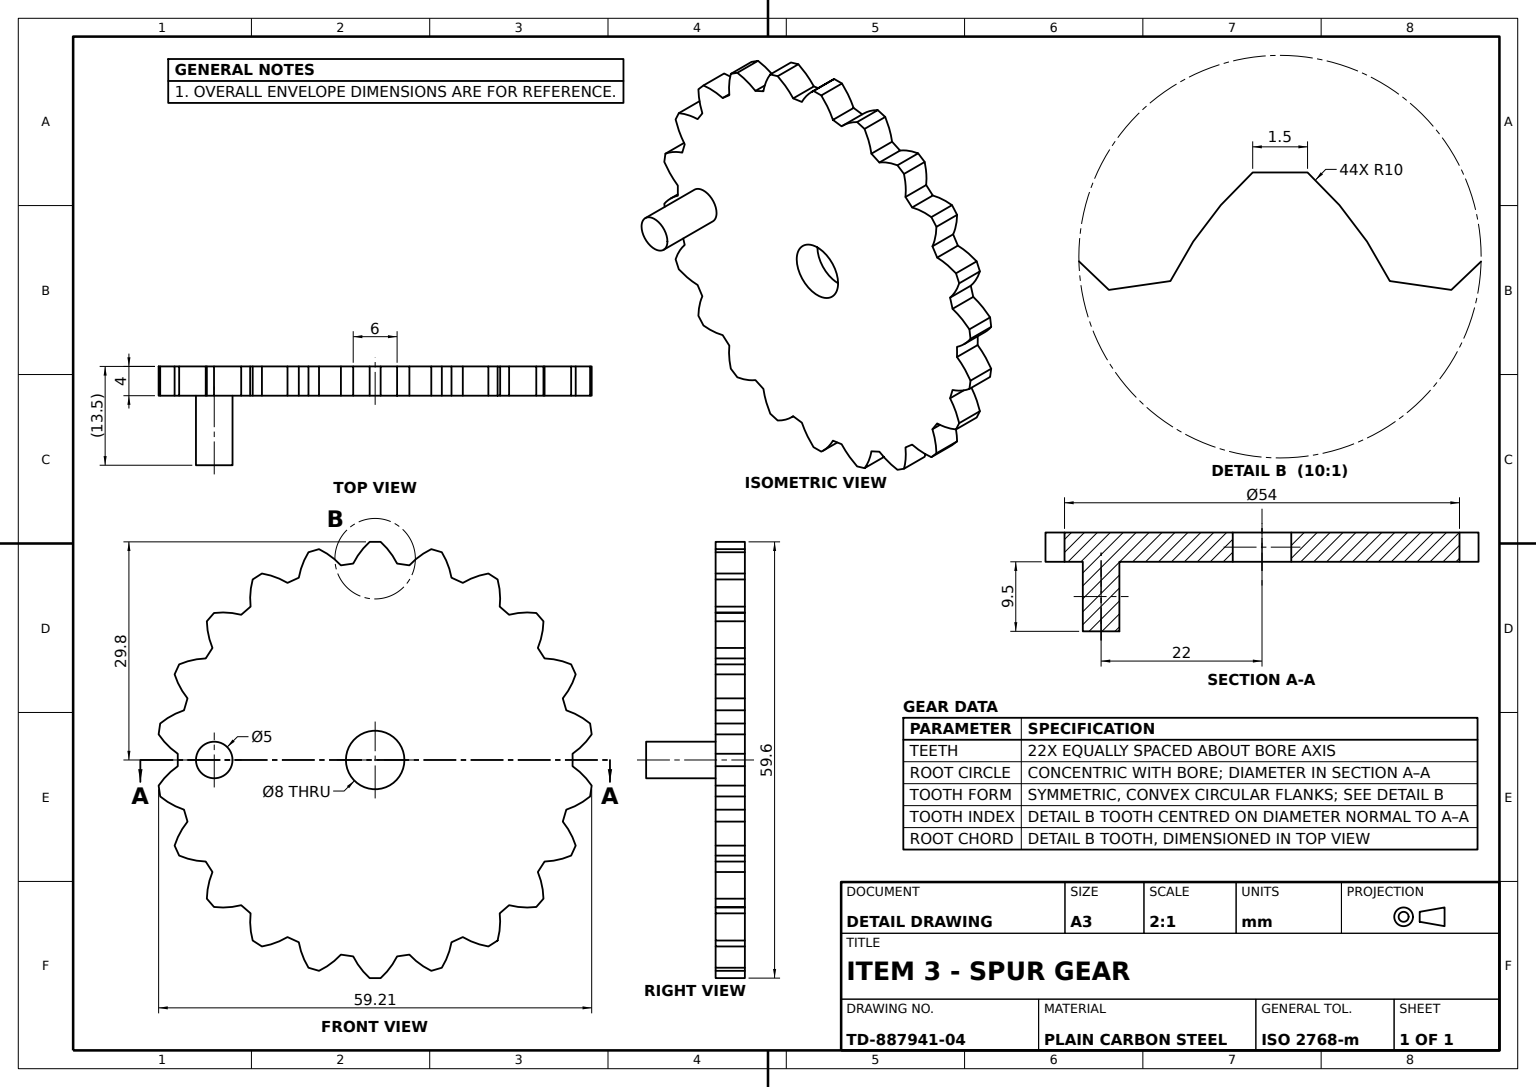
solid
v1 (-3,-26.832816,-4)
v2 (-3,-26.832816,0)
e1 v1 v2 LINE
v3 (-0.75,-29.8,-4)
e2 v3 v1 CIRCLE(AX(P(5.95383,-22.379848,-4),D(0,0,-1),D(1,0,0)),10)
v4 (-0.75,-29.8,0)
e3 v3 v4 LINE
e4 v4 v2 CIRCLE(AX(P(5.95383,-22.379848,0),D(0,0,-1),D(1,0,0)),10)
face CYL(AX(P(5.95383,-22.379848,-4),D(0,0,1),D(1,0,0)),10) [-e1 -e2 e3 e4]
v5 (-15.480156,-25.474836,0)
v6 (-16.742037,-24.663875,0)
e5 v5 v6 LINE
v7 (-16.742037,-24.663875,-4)
e6 v7 v6 LINE
v8 (-15.480156,-25.474836,-4)
e7 v8 v7 LINE
e8 v8 v5 LINE
face PLANE(AX(P(-16.111096,-25.069355,-4),D(0.540640817,0.841253533,0),D(-0.841253533,0.540640817,0))) rev [e5 -e6 -e7 e8]
v9 (-0.75,29.8,0)
v10 (-3,26.832816,0)
e9 v9 v10 CIRCLE(AX(P(5.95383,22.379848,0),D(0,0,1),D(1,0,0)),10)
v11 (-0.75,29.8,-4)
e10 v11 v9 LINE
v12 (-3,26.832816,-4)
e11 v11 v12 CIRCLE(AX(P(5.95383,22.379848,-4),D(0,0,1),D(1,0,0)),10)
e12 v12 v10 LINE
face CYL(AX(P(5.95383,22.379848,-4),D(0,0,1),D(1,0,0)),10) [-e9 -e10 e11 e12]
v13 (22.030192,20.081662,0)
v14 (23.012483,18.948038,0)
e13 v13 v14 LINE
v15 (23.012483,18.948038,-4)
e14 v15 v14 LINE
v16 (22.030192,20.081662,-4)
e15 v16 v15 LINE
e16 v16 v13 LINE
face PLANE(AX(P(22.521337,19.51485,-4),D(-0.755749574,-0.654860734,0),D(0.654860734,-0.755749574,0))) rev [e13 -e14 -e15 e16]
v17 (-23.012483,18.948038,-4)
v18 (-22.243471,15.304509,-4)
e17 v17 v18 CIRCLE(AX(P(-13.014631,19.155288,-4),D(0,0,1),D(1,0,0)),10)
v19 (-22.243471,15.304509,0)
e18 v18 v19 LINE
v20 (-23.012483,18.948038,0)
e19 v20 v19 CIRCLE(AX(P(-13.014631,19.155288,0),D(0,0,1),D(1,0,0)),10)
e20 v17 v20 LINE
face CYL(AX(P(-13.014631,19.155288,-4),D(0,0,1),D(1,0,0)),10) [e17 e18 -e19 -e20]
v21 (-7.67601,28.80419,0)
v22 (-4.681199,26.591096,0)
e21 v21 v22 CIRCLE(AX(P(-12.01779,19.795919,0),D(0,0,-1),D(1,0,0)),10)
v23 (-4.681199,26.591096,-4)
e22 v23 v22 LINE
v24 (-7.67601,28.80419,-4)
e23 v24 v23 CIRCLE(AX(P(-12.01779,19.795919,-4),D(0,0,-1),D(1,0,0)),10)
e24 v24 v21 LINE
face CYL(AX(P(-12.01779,19.795919,-4),D(0,0,1),D(1,0,0)),10) [e21 -e22 -e23 e24]
v25 (-19.5,0,9.5)
v26 (-19.5,0,0)
e25 v25 v26 LINE
v27 (-24.5,0,9.5)
e26 v27 v25 CIRCLE(AX(P(-22,0,9.5),D(0,0,1),D(1,0,0)),2.5)
v28 (-24.5,0,0)
e27 v27 v28 LINE
e28 v28 v26 CIRCLE(AX(P(-22,0,0),D(0,0,1),D(1,0,0)),2.5)
face CYL(AX(P(-22,0,9.5),D(0,0,-1),D(-1,0,0)),2.5) [-e25 -e26 e27 e28]
v29 (-15.480156,25.474836,-4)
v30 (-15.480156,25.474836,0)
e29 v29 v30 LINE
v31 (-11.983155,24.195123,0)
e30 v30 v31 CIRCLE(AX(P(-17.10814,15.608242,0),D(0,0,-1),D(1,0,0)),10)
v32 (-11.983155,24.195123,-4)
e31 v32 v31 LINE
e32 v29 v32 CIRCLE(AX(P(-17.10814,15.608242,-4),D(0,0,-1),D(1,0,0)),10)
face CYL(AX(P(-17.10814,15.608242,-4),D(0,0,1),D(1,0,0)),10) [e29 e30 -e31 -e32]
v33 (10.438157,24.9007,-4)
v34 (10.438157,24.9007,0)
e33 v33 v34 LINE
v35 (11.983155,24.195123,0)
e34 v35 v34 CIRCLE(AX(P(0,0,0),D(0,0,1),D(1,0,0)),27)
v36 (11.983155,24.195123,-4)
e35 v36 v35 LINE
e36 v36 v33 CIRCLE(AX(P(0,0,-4),D(0,0,1),D(1,0,0)),27)
face CYL(AX(P(0,0,-4),D(0,0,1),D(1,0,0)),27) [e33 -e34 -e35 e36]
v37 (23.012483,-18.948038,-4)
v38 (22.243471,-15.304509,-4)
e37 v37 v38 CIRCLE(AX(P(13.014631,-19.155288,-4),D(0,0,1),D(1,0,0)),10)
v39 (22.243471,-15.304509,0)
e38 v38 v39 LINE
v40 (23.012483,-18.948038,0)
e39 v40 v39 CIRCLE(AX(P(13.014631,-19.155288,0),D(0,0,1),D(1,0,0)),10)
e40 v37 v40 LINE
face CYL(AX(P(13.014631,-19.155288,-4),D(0,0,1),D(1,0,0)),10) [e37 e38 -e39 -e40]
v41 (-26.986641,-0.849244,-4)
v42 (-26.986641,-0.849244,0)
e41 v41 v42 LINE
v43 (-29.603415,-3.498616,-4)
e42 v43 v41 CIRCLE(AX(P(-21.304735,-9.078213,-4),D(0,0,-1),D(1,0,0)),10)
v44 (-29.603415,-3.498616,0)
e43 v43 v44 LINE
e44 v44 v42 CIRCLE(AX(P(-21.304735,-9.078213,0),D(0,0,-1),D(1,0,0)),10)
face CYL(AX(P(-21.304735,-9.078213,-4),D(0,0,1),D(1,0,0)),10) [-e41 -e42 e43 e44]
v45 (-26.795472,-13.061591,0)
v46 (-27.418595,-11.697143,0)
e45 v45 v46 LINE
v47 (-27.418595,-11.697143,-4)
e46 v47 v46 LINE
v48 (-26.795472,-13.061591,-4)
e47 v48 v47 LINE
e48 v48 v45 LINE
face PLANE(AX(P(-27.107033,-12.379367,-4),D(0.909631995,0.415415013,0),D(-0.415415013,0.909631995,0))) rev [e45 -e46 -e47 e48]
e49 v26 v28 CIRCLE(AX(P(-22,0,0),D(0,0,1),D(1,0,0)),2.5)
e50 v25 v27 CIRCLE(AX(P(-22,0,9.5),D(0,0,1),D(1,0,0)),2.5)
face CYL(AX(P(-22,0,9.5),D(0,0,-1),D(-1,0,0)),2.5) [e25 e49 -e27 -e50]
v49 (7.67601,-28.80419,-4)
v50 (7.67601,-28.80419,0)
e51 v49 v50 LINE
v51 (4.681199,-26.591096,0)
e52 v50 v51 CIRCLE(AX(P(12.01779,-19.795919,0),D(0,0,-1),D(1,0,0)),10)
v52 (4.681199,-26.591096,-4)
e53 v52 v51 LINE
e54 v49 v52 CIRCLE(AX(P(12.01779,-19.795919,-4),D(0,0,-1),D(1,0,0)),10)
face CYL(AX(P(12.01779,-19.795919,-4),D(0,0,1),D(1,0,0)),10) [e51 e52 -e53 -e54]
v53 (29.603415,-3.498616,0)
v54 (29.389943,-4.983348,0)
e55 v53 v54 LINE
v55 (29.389943,-4.983348,-4)
e56 v55 v54 LINE
v56 (29.603415,-3.498616,-4)
e57 v56 v55 LINE
e58 v56 v53 LINE
face PLANE(AX(P(29.496679,-4.240982,-4),D(-0.989821442,0.142314838,0),D(-0.142314838,-0.989821442,0))) rev [e55 -e56 -e57 e58]
v57 (-22.030192,-20.081662,0)
v58 (-18.314307,-19.839006,0)
e59 v57 v58 CIRCLE(AX(P(-20.81249,-10.156079,0),D(0,0,1),D(1,0,0)),10)
v59 (-22.030192,-20.081662,-4)
e60 v59 v57 LINE
v60 (-18.314307,-19.839006,-4)
e61 v59 v60 CIRCLE(AX(P(-20.81249,-10.156079,-4),D(0,0,1),D(1,0,0)),10)
e62 v60 v58 LINE
face CYL(AX(P(-20.81249,-10.156079,-4),D(0,0,1),D(1,0,0)),10) [-e59 -e60 e61 e62]
v61 (22.030192,-20.081662,-4)
v62 (18.314307,-19.839006,-4)
e63 v61 v62 CIRCLE(AX(P(20.81249,-10.156079,-4),D(0,0,-1),D(1,0,0)),10)
v63 (22.030192,-20.081662,0)
e64 v61 v63 LINE
v64 (18.314307,-19.839006,0)
e65 v63 v64 CIRCLE(AX(P(20.81249,-10.156079,0),D(0,0,-1),D(1,0,0)),10)
e66 v62 v64 LINE
face CYL(AX(P(20.81249,-10.156079,-4),D(0,0,1),D(1,0,0)),10) [-e63 e64 e65 -e66]
v65 (27,0,-4)
v66 (26.986641,0.849244,-4)
e67 v65 v66 CIRCLE(AX(P(0,0,-4),D(0,0,1),D(1,0,0)),27)
v67 (26.986641,0.849244,0)
e68 v66 v67 LINE
v68 (27,0,0)
e69 v68 v67 CIRCLE(AX(P(0,0,0),D(0,0,1),D(1,0,0)),27)
e70 v65 v68 LINE
face CYL(AX(P(0,0,-4),D(0,0,1),D(1,0,0)),27) [e67 e68 -e69 -e70]
v69 (-22.030192,20.081662,-4)
e71 v17 v69 LINE
v70 (-22.030192,20.081662,0)
e72 v20 v70 LINE
e73 v69 v70 LINE
face PLANE(AX(P(-22.521337,19.51485,-4),D(0.755749574,-0.654860734,0),D(0.654860734,0.755749574,0))) rev [-e71 e20 e72 -e73]
v71 (27.418595,11.697143,-4)
v72 (27.418595,11.697143,0)
e74 v71 v72 LINE
v73 (25.654233,8.417859,0)
e75 v72 v73 CIRCLE(AX(P(17.884115,14.712719,0),D(0,0,-1),D(1,0,0)),10)
v74 (25.654233,8.417859,-4)
e76 v74 v73 LINE
e77 v71 v74 CIRCLE(AX(P(17.884115,14.712719,-4),D(0,0,-1),D(1,0,0)),10)
face CYL(AX(P(17.884115,14.712719,-4),D(0,0,1),D(1,0,0)),10) [e74 e75 -e76 -e77]
v75 (-17.030676,-20.951279,-4)
e78 v60 v75 CIRCLE(AX(P(0,0,-4),D(0,0,1),D(1,0,0)),27)
v76 (-17.030676,-20.951279,0)
e79 v75 v76 LINE
e80 v58 v76 CIRCLE(AX(P(0,0,0),D(0,0,1),D(1,0,0)),27)
face CYL(AX(P(0,0,-4),D(0,0,1),D(1,0,0)),27) [-e62 e78 e79 -e80]
v77 (-16.742037,24.663875,-4)
v78 (-16.742037,24.663875,0)
e81 v77 v78 LINE
e82 v78 v30 LINE
e83 v77 v29 LINE
face PLANE(AX(P(-16.111096,25.069355,-4),D(0.540640817,-0.841253533,0),D(0.841253533,0.540640817,0))) rev [e81 e82 -e29 -e83]
v79 (-26.795472,13.061591,-4)
v80 (-23.161743,13.87565,-4)
e84 v79 v80 CIRCLE(AX(P(-22.830736,3.88113,-4),D(0,0,-1),D(1,0,0)),10)
v81 (-26.795472,13.061591,0)
e85 v79 v81 LINE
v82 (-23.161743,13.87565,0)
e86 v81 v82 CIRCLE(AX(P(-22.830736,3.88113,0),D(0,0,-1),D(1,0,0)),10)
e87 v80 v82 LINE
face CYL(AX(P(-22.830736,3.88113,-4),D(0,0,1),D(1,0,0)),10) [-e84 e85 e86 -e87]
v83 (4.681199,26.591096,-4)
v84 (3,26.832816,-4)
e88 v83 v84 CIRCLE(AX(P(0,0,-4),D(0,0,1),D(1,0,0)),27)
v85 (3,26.832816,0)
e89 v84 v85 LINE
v86 (4.681199,26.591096,0)
e90 v86 v85 CIRCLE(AX(P(0,0,0),D(0,0,1),D(1,0,0)),27)
e91 v83 v86 LINE
face CYL(AX(P(0,0,-4),D(0,0,1),D(1,0,0)),27) [e88 e89 -e90 -e91]
v87 (23.161743,13.87565,-4)
v88 (23.161743,13.87565,0)
e92 v87 v88 LINE
v89 (26.795472,13.061591,0)
e93 v89 v88 CIRCLE(AX(P(22.830736,3.88113,0),D(0,0,1),D(1,0,0)),10)
v90 (26.795472,13.061591,-4)
e94 v90 v89 LINE
e95 v90 v87 CIRCLE(AX(P(22.830736,3.88113,-4),D(0,0,1),D(1,0,0)),10)
face CYL(AX(P(22.830736,3.88113,-4),D(0,0,1),D(1,0,0)),10) [e92 -e93 -e94 e95]
v91 (-29.389943,-4.983348,0)
v92 (-26.132752,-6.788172,0)
e96 v91 v92 CIRCLE(AX(P(-22.999371,2.708244,0),D(0,0,1),D(1,0,0)),10)
v93 (-29.389943,-4.983348,-4)
e97 v93 v91 LINE
v94 (-26.132752,-6.788172,-4)
e98 v93 v94 CIRCLE(AX(P(-22.999371,2.708244,-4),D(0,0,1),D(1,0,0)),10)
e99 v94 v92 LINE
face CYL(AX(P(-22.999371,2.708244,-4),D(0,0,1),D(1,0,0)),10) [-e96 -e97 e98 e99]
v95 (7.67601,28.80419,-4)
v96 (9.11525,28.381591,-4)
e100 v95 v96 LINE
v97 (7.67601,28.80419,0)
e101 v95 v97 LINE
v98 (9.11525,28.381591,0)
e102 v97 v98 LINE
e103 v96 v98 LINE
face PLANE(AX(P(8.39563,28.592891,-4),D(-0.281732557,-0.959492974,0),D(0.959492974,-0.281732557,0))) rev [-e100 e101 e102 -e103]
v99 (-26.986641,0.849244,0)
e104 v99 v42 CIRCLE(AX(P(0,0,0),D(0,0,1),D(1,0,0)),27)
v100 (-26.986641,0.849244,-4)
e105 v100 v99 LINE
e106 v100 v41 CIRCLE(AX(P(0,0,-4),D(0,0,1),D(1,0,0)),27)
face CYL(AX(P(0,0,-4),D(0,0,1),D(1,0,0)),27) [-e104 -e105 e106 e41]
v101 (-17.030676,20.951279,-4)
v102 (-18.314307,19.839006,-4)
e107 v101 v102 CIRCLE(AX(P(0,0,-4),D(0,0,1),D(1,0,0)),27)
v103 (-18.314307,19.839006,0)
e108 v102 v103 LINE
v104 (-17.030676,20.951279,0)
e109 v104 v103 CIRCLE(AX(P(0,0,0),D(0,0,1),D(1,0,0)),27)
e110 v101 v104 LINE
face CYL(AX(P(0,0,-4),D(0,0,1),D(1,0,0)),27) [e107 e108 -e109 -e110]
v105 (15.480156,-25.474836,-4)
v106 (15.480156,-25.474836,0)
e111 v105 v106 LINE
v107 (16.742037,-24.663875,-4)
e112 v107 v105 LINE
v108 (16.742037,-24.663875,0)
e113 v107 v108 LINE
e114 v108 v106 LINE
face PLANE(AX(P(16.111096,-25.069355,-4),D(-0.540640817,0.841253533,0),D(-0.841253533,-0.540640817,0))) rev [-e111 -e112 e113 e114]
v109 (26.986641,-0.849244,-4)
e115 v56 v109 CIRCLE(AX(P(21.304735,-9.078213,-4),D(0,0,1),D(1,0,0)),10)
v110 (26.986641,-0.849244,0)
e116 v109 v110 LINE
e117 v53 v110 CIRCLE(AX(P(21.304735,-9.078213,0),D(0,0,1),D(1,0,0)),10)
face CYL(AX(P(21.304735,-9.078213,-4),D(0,0,1),D(1,0,0)),10) [e115 e116 -e117 -e58]
v111 (29.603415,3.498616,-4)
v112 (29.603415,3.498616,0)
e118 v111 v112 LINE
v113 (29.389943,4.983348,-4)
e119 v113 v111 LINE
v114 (29.389943,4.983348,0)
e120 v113 v114 LINE
e121 v114 v112 LINE
face PLANE(AX(P(29.496679,4.240982,-4),D(-0.989821442,-0.142314838,0),D(0.142314838,-0.989821442,0))) rev [-e118 -e119 e120 e121]
v115 (0.75,-29.8,-4)
e122 v115 v3 LINE
v116 (0.75,-29.8,0)
e123 v115 v116 LINE
e124 v116 v4 LINE
face PLANE(AX(P(0,-29.8,-4),D(0,1,0),D(0,0,1))) rev [-e122 e123 e124 -e3]
v117 (17.030676,-20.951279,-4)
v118 (17.030676,-20.951279,0)
e125 v117 v118 LINE
e126 v117 v62 CIRCLE(AX(P(0,0,-4),D(0,0,1),D(1,0,0)),27)
e127 v118 v64 CIRCLE(AX(P(0,0,0),D(0,0,1),D(1,0,0)),27)
face CYL(AX(P(0,0,-4),D(0,0,1),D(1,0,0)),27) [-e125 e126 e66 -e127]
v119 (27.418595,-11.697143,-4)
v120 (27.418595,-11.697143,0)
e128 v119 v120 LINE
v121 (25.654233,-8.417859,-4)
e129 v119 v121 CIRCLE(AX(P(17.884115,-14.712719,-4),D(0,0,1),D(1,0,0)),10)
v122 (25.654233,-8.417859,0)
e130 v121 v122 LINE
e131 v120 v122 CIRCLE(AX(P(17.884115,-14.712719,0),D(0,0,1),D(1,0,0)),10)
face CYL(AX(P(17.884115,-14.712719,-4),D(0,0,1),D(1,0,0)),10) [-e128 e129 e130 -e131]
e132 v109 v65 CIRCLE(AX(P(0,0,-4),D(0,0,1),D(1,0,0)),27)
e133 v110 v68 CIRCLE(AX(P(0,0,0),D(0,0,1),D(1,0,0)),27)
face CYL(AX(P(0,0,-4),D(0,0,1),D(1,0,0)),27) [e132 e70 -e133 -e116]
e134 v10 v22 CIRCLE(AX(P(0,0,0),D(0,0,1),D(1,0,0)),27)
v123 (-9.11525,28.381591,0)
e135 v123 v21 LINE
v124 (-10.438157,24.9007,0)
e136 v123 v124 CIRCLE(AX(P(-0.592473,23.150694,0),D(0,0,1),D(1,0,0)),10)
e137 v124 v31 CIRCLE(AX(P(0,0,0),D(0,0,1),D(1,0,0)),27)
e138 v78 v104 CIRCLE(AX(P(-7.090778,22.04601,0),D(0,0,1),D(1,0,0)),10)
e139 v70 v103 CIRCLE(AX(P(-20.81249,10.156079,0),D(0,0,-1),D(1,0,0)),10)
e140 v19 v82 CIRCLE(AX(P(0,0,0),D(0,0,1),D(1,0,0)),27)
v125 (-27.418595,11.697143,0)
e141 v125 v81 LINE
v126 (-25.654233,8.417859,0)
e142 v125 v126 CIRCLE(AX(P(-17.884115,14.712719,0),D(0,0,1),D(1,0,0)),10)
v127 (-26.132752,6.788172,0)
e143 v126 v127 CIRCLE(AX(P(0,0,0),D(0,0,1),D(1,0,0)),27)
v128 (-29.389943,4.983348,0)
e144 v128 v127 CIRCLE(AX(P(-22.999371,-2.708244,0),D(0,0,-1),D(1,0,0)),10)
v129 (-29.603415,3.498616,0)
e145 v129 v128 LINE
e146 v129 v99 CIRCLE(AX(P(-21.304735,9.078213,0),D(0,0,1),D(1,0,0)),10)
e147 v91 v44 LINE
v130 (-25.654233,-8.417859,0)
e148 v92 v130 CIRCLE(AX(P(0,0,0),D(0,0,1),D(1,0,0)),27)
e149 v46 v130 CIRCLE(AX(P(-17.884115,-14.712719,0),D(0,0,-1),D(1,0,0)),10)
v131 (-23.161743,-13.87565,0)
e150 v45 v131 CIRCLE(AX(P(-22.830736,-3.88113,0),D(0,0,1),D(1,0,0)),10)
v132 (-22.243471,-15.304509,0)
e151 v131 v132 CIRCLE(AX(P(0,0,0),D(0,0,1),D(1,0,0)),27)
v133 (-23.012483,-18.948038,0)
e152 v133 v132 CIRCLE(AX(P(-13.014631,-19.155288,0),D(0,0,-1),D(1,0,0)),10)
e153 v57 v133 LINE
e154 v6 v76 CIRCLE(AX(P(-7.090778,-22.04601,0),D(0,0,-1),D(1,0,0)),10)
v134 (-11.983155,-24.195123,0)
e155 v5 v134 CIRCLE(AX(P(-17.10814,-15.608242,0),D(0,0,1),D(1,0,0)),10)
v135 (-10.438157,-24.9007,0)
e156 v134 v135 CIRCLE(AX(P(0,0,0),D(0,0,1),D(1,0,0)),27)
v136 (-9.11525,-28.381591,0)
e157 v136 v135 CIRCLE(AX(P(-0.592473,-23.150694,0),D(0,0,-1),D(1,0,0)),10)
v137 (-7.67601,-28.80419,0)
e158 v137 v136 LINE
v138 (-4.681199,-26.591096,0)
e159 v137 v138 CIRCLE(AX(P(-12.01779,-19.795919,0),D(0,0,1),D(1,0,0)),10)
e160 v138 v2 CIRCLE(AX(P(0,0,0),D(0,0,1),D(1,0,0)),27)
v139 (3,-26.832816,0)
e161 v116 v139 CIRCLE(AX(P(-5.95383,-22.379848,0),D(0,0,1),D(1,0,0)),10)
e162 v139 v51 CIRCLE(AX(P(0,0,0),D(0,0,1),D(1,0,0)),27)
v140 (9.11525,-28.381591,0)
e163 v140 v50 LINE
v141 (10.438157,-24.9007,0)
e164 v140 v141 CIRCLE(AX(P(0.592473,-23.150694,0),D(0,0,1),D(1,0,0)),10)
v142 (11.983155,-24.195123,0)
e165 v141 v142 CIRCLE(AX(P(0,0,0),D(0,0,1),D(1,0,0)),27)
e166 v106 v142 CIRCLE(AX(P(17.10814,-15.608242,0),D(0,0,-1),D(1,0,0)),10)
v143 (17.090778,-22.04601,0)
e167 v108 v143 CIRCLE(AX(P(7.090778,-22.04601,0),D(0,0,1),D(1,0,0)),10)
e168 v143 v118 CIRCLE(AX(P(7.090778,-22.04601,0),D(0,0,1),D(1,0,0)),10)
e169 v40 v63 LINE
v144 (23.161743,-13.87565,0)
e170 v39 v144 CIRCLE(AX(P(0,0,0),D(0,0,1),D(1,0,0)),27)
v145 (26.795472,-13.061591,0)
e171 v145 v144 CIRCLE(AX(P(22.830736,-3.88113,0),D(0,0,-1),D(1,0,0)),10)
e172 v120 v145 LINE
v146 (26.132752,-6.788172,0)
e173 v122 v146 CIRCLE(AX(P(0,0,0),D(0,0,1),D(1,0,0)),27)
e174 v54 v146 CIRCLE(AX(P(22.999371,2.708244,0),D(0,0,-1),D(1,0,0)),10)
e175 v112 v67 CIRCLE(AX(P(21.304735,9.078213,0),D(0,0,-1),D(1,0,0)),10)
v147 (26.132752,6.788172,0)
e176 v114 v147 CIRCLE(AX(P(22.999371,-2.708244,0),D(0,0,1),D(1,0,0)),10)
e177 v147 v73 CIRCLE(AX(P(0,0,0),D(0,0,1),D(1,0,0)),27)
e178 v89 v72 LINE
v148 (22.243471,15.304509,0)
e179 v88 v148 CIRCLE(AX(P(0,0,0),D(0,0,1),D(1,0,0)),27)
e180 v14 v148 CIRCLE(AX(P(13.014631,19.155288,0),D(0,0,-1),D(1,0,0)),10)
v149 (18.314307,19.839006,0)
e181 v13 v149 CIRCLE(AX(P(20.81249,10.156079,0),D(0,0,1),D(1,0,0)),10)
v150 (17.030676,20.951279,0)
e182 v149 v150 CIRCLE(AX(P(0,0,0),D(0,0,1),D(1,0,0)),27)
v151 (17.090778,22.04601,0)
e183 v151 v150 CIRCLE(AX(P(7.090778,22.04601,0),D(0,0,-1),D(1,0,0)),10)
v152 (16.742037,24.663875,0)
e184 v152 v151 CIRCLE(AX(P(7.090778,22.04601,0),D(0,0,-1),D(1,0,0)),10)
v153 (15.480156,25.474836,0)
e185 v153 v152 LINE
e186 v153 v35 CIRCLE(AX(P(17.10814,15.608242,0),D(0,0,1),D(1,0,0)),10)
e187 v98 v34 CIRCLE(AX(P(0.592473,23.150694,0),D(0,0,-1),D(1,0,0)),10)
e188 v97 v86 CIRCLE(AX(P(12.01779,19.795919,0),D(0,0,1),D(1,0,0)),10)
v154 (0.75,29.8,0)
e189 v154 v85 CIRCLE(AX(P(-5.95383,22.379848,0),D(0,0,-1),D(1,0,0)),10)
e190 v9 v154 LINE
v155 (-4,0,0)
v156 (4,0,0)
e191 v155 v156 CIRCLE(AX(P(0,0,0),D(0,0,1),D(1,0,0)),4)
e192 v156 v155 CIRCLE(AX(P(0,0,0),D(0,0,1),D(1,0,0)),4)
face PLANE(AX(P(0,0,0),D(0,0,1),D(1,0,0))) [e9 e134 -e21 -e135 e136 e137 -e30 -e82 e138 e109 -e139 -e72 e19 e140 -e86 -e141 e142 e143 -e144 -e145 e146 e104 -e44 -e147 e96 e148 -e149 -e45 e150 e151 -e152 -e153 e59 e80 -e154 -e5 e155 e156 -e157 -e158 e159 e160 -e4 -e124 e161 e162 -e52 -e163 e164 e165 -e166 -e114 e167 e168 e127 -e65 -e169 e39 e170 -e171 -e172 e131 e173 -e174 -e55 e117 e133 e69 -e175 -e121 e176 e177 -e75 -e178 e93 e179 -e180 -e13 e181 e182 -e183 -e184 -e185 e186 e34 -e187 -e102 e188 e90 -e189 -e190] [-e191 -e192] [-e28 -e49]
e193 v18 v80 CIRCLE(AX(P(0,0,-4),D(0,0,1),D(1,0,0)),27)
face CYL(AX(P(0,0,-4),D(0,0,1),D(1,0,0)),27) [e193 e87 -e140 -e18]
v157 (-9.11525,28.381591,-4)
e194 v157 v123 LINE
v158 (-10.438157,24.9007,-4)
e195 v157 v158 CIRCLE(AX(P(-0.592473,23.150694,-4),D(0,0,1),D(1,0,0)),10)
e196 v158 v124 LINE
face CYL(AX(P(-0.592473,23.150694,-4),D(0,0,1),D(1,0,0)),10) [-e194 e195 e196 -e136]
v159 (-7.67601,-28.80419,-4)
v160 (-4.681199,-26.591096,-4)
e197 v159 v160 CIRCLE(AX(P(-12.01779,-19.795919,-4),D(0,0,1),D(1,0,0)),10)
e198 v160 v138 LINE
e199 v159 v137 LINE
face CYL(AX(P(-12.01779,-19.795919,-4),D(0,0,1),D(1,0,0)),10) [e197 e198 -e159 -e199]
v161 (0.75,29.8,-4)
e200 v161 v154 LINE
e201 v11 v161 LINE
face PLANE(AX(P(0,29.8,-4),D(0,-1,0),D(0,0,-1))) rev [-e200 -e201 e10 e190]
e202 v90 v71 LINE
face PLANE(AX(P(27.107033,12.379367,-4),D(-0.909631995,-0.415415013,0),D(0.415415013,-0.909631995,0))) rev [-e74 -e202 e94 e178]
v162 (9.11525,-28.381591,-4)
e203 v162 v140 LINE
e204 v162 v49 LINE
face PLANE(AX(P(8.39563,-28.592891,-4),D(-0.281732557,0.959492974,0),D(-0.959492974,-0.281732557,0))) rev [e203 e163 -e51 -e204]
v163 (26.795472,-13.061591,-4)
e205 v163 v145 LINE
e206 v119 v163 LINE
face PLANE(AX(P(27.107033,-12.379367,-4),D(-0.909631995,0.415415013,0),D(-0.415415013,-0.909631995,0))) rev [e172 -e205 -e206 e128]
v164 (-29.389943,4.983348,-4)
e207 v164 v128 LINE
v165 (-29.603415,3.498616,-4)
e208 v165 v164 LINE
e209 v165 v129 LINE
face PLANE(AX(P(-29.496679,4.240982,-4),D(0.989821442,-0.142314838,0),D(0.142314838,0.989821442,0))) rev [-e207 -e208 e209 e145]
v166 (-25.654233,8.417859,-4)
e210 v166 v126 LINE
v167 (-27.418595,11.697143,-4)
e211 v167 v125 LINE
e212 v167 v166 CIRCLE(AX(P(-17.884115,14.712719,-4),D(0,0,1),D(1,0,0)),10)
face CYL(AX(P(-17.884115,14.712719,-4),D(0,0,1),D(1,0,0)),10) [e210 -e142 -e211 e212]
v168 (11.983155,-24.195123,-4)
e213 v168 v142 LINE
e214 v105 v168 CIRCLE(AX(P(17.10814,-15.608242,-4),D(0,0,-1),D(1,0,0)),10)
face CYL(AX(P(17.10814,-15.608242,-4),D(0,0,1),D(1,0,0)),10) [e111 e166 -e213 -e214]
v169 (4,0,-4)
v170 (-4,0,-4)
e215 v169 v170 CIRCLE(AX(P(0,0,-4),D(0,0,1),D(1,0,0)),4)
e216 v170 v169 CIRCLE(AX(P(0,0,-4),D(0,0,1),D(1,0,0)),4)
v171 (-26.132752,6.788172,-4)
e217 v164 v171 CIRCLE(AX(P(-22.999371,-2.708244,-4),D(0,0,-1),D(1,0,0)),10)
e218 v166 v171 CIRCLE(AX(P(0,0,-4),D(0,0,1),D(1,0,0)),27)
e219 v167 v79 LINE
e220 v69 v102 CIRCLE(AX(P(-20.81249,10.156079,-4),D(0,0,-1),D(1,0,0)),10)
e221 v77 v101 CIRCLE(AX(P(-7.090778,22.04601,-4),D(0,0,1),D(1,0,0)),10)
e222 v158 v32 CIRCLE(AX(P(0,0,-4),D(0,0,1),D(1,0,0)),27)
e223 v157 v24 LINE
e224 v12 v23 CIRCLE(AX(P(0,0,-4),D(0,0,1),D(1,0,0)),27)
e225 v161 v84 CIRCLE(AX(P(-5.95383,22.379848,-4),D(0,0,-1),D(1,0,0)),10)
e226 v95 v83 CIRCLE(AX(P(12.01779,19.795919,-4),D(0,0,1),D(1,0,0)),10)
e227 v96 v33 CIRCLE(AX(P(0.592473,23.150694,-4),D(0,0,-1),D(1,0,0)),10)
v172 (15.480156,25.474836,-4)
e228 v172 v36 CIRCLE(AX(P(17.10814,15.608242,-4),D(0,0,1),D(1,0,0)),10)
v173 (16.742037,24.663875,-4)
e229 v172 v173 LINE
v174 (17.090778,22.04601,-4)
e230 v173 v174 CIRCLE(AX(P(7.090778,22.04601,-4),D(0,0,-1),D(1,0,0)),10)
v175 (17.030676,20.951279,-4)
e231 v174 v175 CIRCLE(AX(P(7.090778,22.04601,-4),D(0,0,-1),D(1,0,0)),10)
v176 (18.314307,19.839006,-4)
e232 v176 v175 CIRCLE(AX(P(0,0,-4),D(0,0,1),D(1,0,0)),27)
e233 v16 v176 CIRCLE(AX(P(20.81249,10.156079,-4),D(0,0,1),D(1,0,0)),10)
v177 (22.243471,15.304509,-4)
e234 v15 v177 CIRCLE(AX(P(13.014631,19.155288,-4),D(0,0,-1),D(1,0,0)),10)
e235 v87 v177 CIRCLE(AX(P(0,0,-4),D(0,0,1),D(1,0,0)),27)
v178 (26.132752,6.788172,-4)
e236 v178 v74 CIRCLE(AX(P(0,0,-4),D(0,0,1),D(1,0,0)),27)
e237 v113 v178 CIRCLE(AX(P(22.999371,-2.708244,-4),D(0,0,1),D(1,0,0)),10)
e238 v111 v66 CIRCLE(AX(P(21.304735,9.078213,-4),D(0,0,-1),D(1,0,0)),10)
v179 (26.132752,-6.788172,-4)
e239 v55 v179 CIRCLE(AX(P(22.999371,2.708244,-4),D(0,0,-1),D(1,0,0)),10)
e240 v121 v179 CIRCLE(AX(P(0,0,-4),D(0,0,1),D(1,0,0)),27)
v180 (23.161743,-13.87565,-4)
e241 v163 v180 CIRCLE(AX(P(22.830736,-3.88113,-4),D(0,0,-1),D(1,0,0)),10)
e242 v38 v180 CIRCLE(AX(P(0,0,-4),D(0,0,1),D(1,0,0)),27)
e243 v37 v61 LINE
v181 (17.090778,-22.04601,-4)
e244 v181 v117 CIRCLE(AX(P(7.090778,-22.04601,-4),D(0,0,1),D(1,0,0)),10)
e245 v107 v181 CIRCLE(AX(P(7.090778,-22.04601,-4),D(0,0,1),D(1,0,0)),10)
v182 (10.438157,-24.9007,-4)
e246 v182 v168 CIRCLE(AX(P(0,0,-4),D(0,0,1),D(1,0,0)),27)
e247 v162 v182 CIRCLE(AX(P(0.592473,-23.150694,-4),D(0,0,1),D(1,0,0)),10)
v183 (3,-26.832816,-4)
e248 v183 v52 CIRCLE(AX(P(0,0,-4),D(0,0,1),D(1,0,0)),27)
e249 v115 v183 CIRCLE(AX(P(-5.95383,-22.379848,-4),D(0,0,1),D(1,0,0)),10)
e250 v160 v1 CIRCLE(AX(P(0,0,-4),D(0,0,1),D(1,0,0)),27)
v184 (-9.11525,-28.381591,-4)
e251 v159 v184 LINE
v185 (-10.438157,-24.9007,-4)
e252 v184 v185 CIRCLE(AX(P(-0.592473,-23.150694,-4),D(0,0,-1),D(1,0,0)),10)
v186 (-11.983155,-24.195123,-4)
e253 v186 v185 CIRCLE(AX(P(0,0,-4),D(0,0,1),D(1,0,0)),27)
e254 v8 v186 CIRCLE(AX(P(-17.10814,-15.608242,-4),D(0,0,1),D(1,0,0)),10)
e255 v7 v75 CIRCLE(AX(P(-7.090778,-22.04601,-4),D(0,0,-1),D(1,0,0)),10)
v187 (-23.012483,-18.948038,-4)
e256 v59 v187 LINE
v188 (-22.243471,-15.304509,-4)
e257 v187 v188 CIRCLE(AX(P(-13.014631,-19.155288,-4),D(0,0,-1),D(1,0,0)),10)
v189 (-23.161743,-13.87565,-4)
e258 v189 v188 CIRCLE(AX(P(0,0,-4),D(0,0,1),D(1,0,0)),27)
e259 v48 v189 CIRCLE(AX(P(-22.830736,-3.88113,-4),D(0,0,1),D(1,0,0)),10)
v190 (-25.654233,-8.417859,-4)
e260 v47 v190 CIRCLE(AX(P(-17.884115,-14.712719,-4),D(0,0,-1),D(1,0,0)),10)
e261 v94 v190 CIRCLE(AX(P(0,0,-4),D(0,0,1),D(1,0,0)),27)
e262 v93 v43 LINE
e263 v165 v100 CIRCLE(AX(P(-21.304735,9.078213,-4),D(0,0,1),D(1,0,0)),10)
face PLANE(AX(P(0,0,-4),D(0,0,1),D(1,0,0))) rev [e215 e216] [e217 -e218 -e212 e219 e84 -e193 -e17 e71 e220 -e107 -e221 e83 e32 -e222 -e195 e223 e23 -e224 -e11 e201 e225 -e88 -e226 e100 e227 -e36 -e228 e229 e230 e231 -e232 -e233 e15 e234 -e235 -e95 e202 e77 -e236 -e237 e119 e238 -e67 -e132 -e115 e57 e239 -e240 -e129 e206 e241 -e242 -e37 e243 e63 -e126 -e244 -e245 e112 e214 -e246 -e247 e204 e54 -e248 -e249 e122 e2 -e250 -e197 e251 e252 -e253 -e254 e7 e255 -e78 -e61 e256 e257 -e258 -e259 e47 e260 -e261 -e98 e262 e42 -e106 -e263 e208]
face PLANE(AX(P(-27.107033,12.379367,-4),D(0.909631995,-0.415415013,0),D(0.415415013,0.909631995,0))) rev [-e219 e211 e141 -e85]
face CYL(AX(P(0,0,-4),D(0,0,1),D(1,0,0)),27) [e1 -e160 -e198 e250]
e264 v170 v155 LINE
e265 v169 v156 LINE
face CYL(AX(P(0,0,-4),D(0,0,1),D(1,0,0)),4) rev [e192 -e264 -e215 e265]
e266 v171 v127 LINE
face CYL(AX(P(-22.999371,-2.708244,-4),D(0,0,1),D(1,0,0)),10) [-e266 -e217 e207 e144]
e267 v176 v149 LINE
face CYL(AX(P(20.81249,10.156079,-4),D(0,0,1),D(1,0,0)),10) [e233 e267 -e181 -e16]
e268 v184 v136 LINE
face PLANE(AX(P(-8.39563,-28.592891,-4),D(0.281732557,0.959492974,0),D(-0.959492974,0.281732557,0))) rev [-e251 e199 e158 -e268]
e269 v181 v143 LINE
face CYL(AX(P(7.090778,-22.04601,-4),D(0,0,1),D(1,0,0)),10) [-e269 e244 e125 -e168]
face CYL(AX(P(-7.090778,-22.04601,-4),D(0,0,1),D(1,0,0)),10) [e6 e154 -e79 -e255]
e270 v186 v134 LINE
face CYL(AX(P(-17.10814,-15.608242,-4),D(0,0,1),D(1,0,0)),10) [-e155 -e8 e254 e270]
e271 v190 v130 LINE
face CYL(AX(P(0,0,-4),D(0,0,1),D(1,0,0)),27) [-e99 e261 e271 -e148]
e272 v185 v135 LINE
face CYL(AX(P(-0.592473,-23.150694,-4),D(0,0,1),D(1,0,0)),10) [e157 -e272 -e252 e268]
face CYL(AX(P(12.01779,19.795919,-4),D(0,0,1),D(1,0,0)),10) [e226 e91 -e188 -e101]
e273 v174 v151 LINE
e274 v173 v152 LINE
face CYL(AX(P(7.090778,22.04601,-4),D(0,0,1),D(1,0,0)),10) [-e273 -e230 e274 e184]
face CYL(AX(P(-5.95383,22.379848,-4),D(0,0,1),D(1,0,0)),10) [-e225 e200 e189 -e89]
face CYL(AX(P(-17.884115,-14.712719,-4),D(0,0,1),D(1,0,0)),10) [e149 -e271 -e260 e46]
face PLANE(AX(P(-8.39563,28.592891,-4),D(0.281732557,-0.959492974,0),D(0.959492974,0.281732557,0))) rev [e194 e135 -e24 -e223]
e275 v175 v150 LINE
face CYL(AX(P(0,0,-4),D(0,0,1),D(1,0,0)),27) [e232 e275 -e182 -e267]
face PLANE(AX(P(-29.496679,-4.240982,-4),D(0.989821442,0.142314838,0),D(-0.142314838,0.989821442,0))) rev [e147 -e43 -e262 e97]
face CYL(AX(P(7.090778,22.04601,-4),D(0,0,1),D(1,0,0)),10) [e273 e183 -e275 -e231]
face CYL(AX(P(0,0,-4),D(0,0,1),D(1,0,0)),27) [e272 -e156 -e270 e253]
face PLANE(AX(P(22.521337,-19.51485,-4),D(-0.755749574,0.654860734,0),D(-0.654860734,-0.755749574,0))) rev [-e64 -e243 e40 e169]
face CYL(AX(P(-21.304735,9.078213,-4),D(0,0,1),D(1,0,0)),10) [e105 -e146 -e209 e263]
face CYL(AX(P(21.304735,9.078213,-4),D(0,0,1),D(1,0,0)),10) [-e238 e118 e175 -e68]
e276 v182 v141 LINE
face CYL(AX(P(0.592473,-23.150694,-4),D(0,0,1),D(1,0,0)),10) [e247 e276 -e164 -e203]
e277 v188 v132 LINE
e278 v187 v133 LINE
face CYL(AX(P(-13.014631,-19.155288,-4),D(0,0,1),D(1,0,0)),10) [e152 -e277 -e257 e278]
e279 v180 v144 LINE
face CYL(AX(P(0,0,-4),D(0,0,1),D(1,0,0)),27) [-e38 e242 e279 -e170]
face CYL(AX(P(-20.81249,10.156079,-4),D(0,0,1),D(1,0,0)),10) [e139 -e108 -e220 e73]
face CYL(AX(P(0,0,-4),D(0,0,1),D(1,0,0)),4) rev [e264 e191 -e265 -e216]
e280 v179 v146 LINE
face CYL(AX(P(0,0,-4),D(0,0,1),D(1,0,0)),27) [-e130 e240 e280 -e173]
face CYL(AX(P(0.592473,23.150694,-4),D(0,0,1),D(1,0,0)),10) [e187 -e33 -e227 e103]
face CYL(AX(P(0,0,-4),D(0,0,1),D(1,0,0)),27) [e246 e213 -e165 -e276]
e281 v178 v147 LINE
face CYL(AX(P(0,0,-4),D(0,0,1),D(1,0,0)),27) [e236 e76 -e177 -e281]
face CYL(AX(P(-7.090778,22.04601,-4),D(0,0,1),D(1,0,0)),10) [e221 e110 -e138 -e81]
e282 v183 v139 LINE
face CYL(AX(P(0,0,-4),D(0,0,1),D(1,0,0)),27) [e53 -e162 -e282 e248]
face CYL(AX(P(7.090778,-22.04601,-4),D(0,0,1),D(1,0,0)),10) [e269 -e167 -e113 e245]
e283 v177 v148 LINE
face CYL(AX(P(0,0,-4),D(0,0,1),D(1,0,0)),27) [-e179 -e92 e235 e283]
e284 v172 v153 LINE
face PLANE(AX(P(16.111096,25.069355,-4),D(-0.540640817,-0.841253533,0),D(0.841253533,-0.540640817,0))) rev [-e229 e284 e185 -e274]
face CYL(AX(P(0,0,-4),D(0,0,1),D(1,0,0)),27) [e22 -e134 -e12 e224]
e285 v189 v131 LINE
face CYL(AX(P(0,0,-4),D(0,0,1),D(1,0,0)),27) [-e285 e258 e277 -e151]
face CYL(AX(P(-5.95383,-22.379848,-4),D(0,0,1),D(1,0,0)),10) [-e123 e249 e282 -e161]
face CYL(AX(P(0,0,-4),D(0,0,1),D(1,0,0)),27) [e218 e266 -e143 -e210]
face PLANE(AX(P(0,0,9.5),D(0,0,1),D(1,0,0))) [e50 e26]
face PLANE(AX(P(-22.521337,-19.51485,-4),D(0.755749574,0.654860734,0),D(-0.654860734,0.755749574,0))) rev [e153 -e278 -e256 e60]
face CYL(AX(P(-22.830736,-3.88113,-4),D(0,0,1),D(1,0,0)),10) [e285 -e150 -e48 e259]
face CYL(AX(P(0,0,-4),D(0,0,1),D(1,0,0)),27) [-e196 e222 e31 -e137]
face CYL(AX(P(13.014631,19.155288,-4),D(0,0,1),D(1,0,0)),10) [e180 -e283 -e234 e14]
face CYL(AX(P(22.830736,-3.88113,-4),D(0,0,1),D(1,0,0)),10) [-e279 -e241 e205 e171]
face CYL(AX(P(22.999371,-2.708244,-4),D(0,0,1),D(1,0,0)),10) [e237 e281 -e176 -e120]
face CYL(AX(P(22.999371,2.708244,-4),D(0,0,1),D(1,0,0)),10) [-e280 -e239 e56 e174]
face CYL(AX(P(17.10814,15.608242,-4),D(0,0,1),D(1,0,0)),10) [e228 e35 -e186 -e284]
